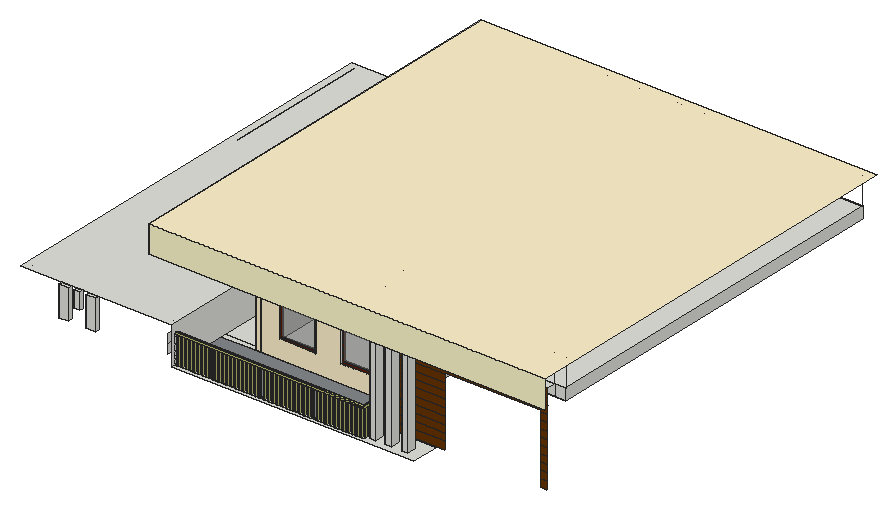
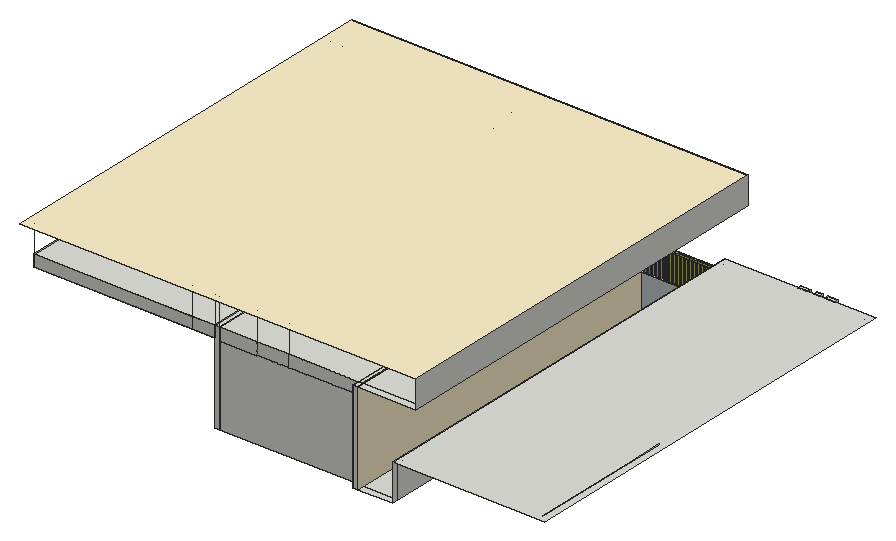
# SketchUp Ruby script. Lengths in inches.
U = 1.inch
M = Sketchup.active_model
def pt(a) = Geom::Point3d.new(a.map { |v| v * U })
def face(e, loops, mat)
  f = e.add_face(loops[0].map { |a| pt(a) })
  loops[1..].each { |l| e.add_face(l.map { |a| pt(a) }).erase! }
  f.material = f.back_material = mat if mat
  f
end
# faces: each face lists its corners as indices into pts; further lists are holes
def faces(e, pts, list, mat = nil) = list.each { |f| face(e, (f[0].is_a?(Array) ? f : [f]).map { |l| l.map { |i| pts[i] } }, mat) }
# xy, xz, yz: faces in a plane at the given z, y or x. An outline is a flat list of corners, or four numbers for a rectangle; further outlines are holes
def ring(l) = l.size == 4 ? [[l[0], l[1]], [l[2], l[1]], [l[2], l[3]], [l[0], l[3]]] : l.each_slice(2).to_a
def flat(e, list, mat, &to3) = list.each { |f| face(e, (f[0].is_a?(Array) ? f : [f]).map { |l| ring(l).map { |u, v| to3.(u, v) } }, mat) }
def xy(e, z, list, mat = nil) = flat(e, list, mat) { |x, y| [x, y, z] }
def xz(e, y, list, mat = nil) = flat(e, list, mat) { |x, z| [x, y, z] }
def yz(e, x, list, mat = nil) = flat(e, list, mat) { |y, z| [x, y, z] }
def lines(e, pts, list) = list.each { |a, b| e.add_line(pt(pts[a]), pt(pts[b])) }
# prism: a flat outline (further loops are holes) pulled along v
def prism(e, loops, v, mat = nil)
  f = face(e, loops, mat); d = Geom::Vector3d.new(v.map { |x| x * U })
  f.pushpull(f.normal.samedirection?(d) ? d.length : -d.length)
end
def box(e, o, s, mat = nil) = prism(e, [[o, [o[0] + s[0], o[1], o[2]], [o[0] + s[0], o[1] + s[1], o[2]], [o[0], o[1] + s[1], o[2]]]], [0, 0, s[2]], mat)
def at(x, y, z, deg = 0) = Geom::Transformation.translation(pt([x, y, z])) * Geom::Transformation.rotation(ORIGIN, Z_AXIS, deg.degrees)
def axes(o, x, y, z) = Geom::Transformation.new([*x, 0, *y, 0, *z, 0, *pt(o).to_a, 1])
def part(name) = M.definitions.add(name)
# library, detail: a bought-in or finely detailed component or shape, given as its bounding box
def library(name, o, s) = part(name).tap { |d| box(d.entities, o, s) }
def detail(e, o, s) = box(e.add_group.entities, o, s)
def put(e, d, t, mat = nil) = e.add_instance(d, t).tap { |i| i.material = mat if mat }
def group(e, t, mat = nil) = e.add_group.tap { |g| g.transformation = t; g.material = mat if mat }.entities
root = M.entities
M.materials.add("[0050_LemonChiffon]").color = [255, 250, 205]
M.materials.add("[Blacktop Old 01]").color = [132, 136, 139]
M.materials.add("[Color B08]").color = [102, 25, 0]
M.materials.add("[Color C08]").color = [102, 51, 0]
M.materials.add("[Color D01]").color = [255, 242, 204]
M.materials.add("[Metal Corrugated Shiny]").color = [193, 193, 113]
M.materials.add("[Translucent Glass Gray]").color = [128, 128, 128]
M.materials["[Translucent Glass Gray]"].alpha = 0.5
c1 = part("Group\#3")
xy(c1.entities,0,[[0,0,43.875,1.8125],[0,1.8125,43.875,3.875]],"[Color B08]")
xy(c1.entities,1.78,[[1.78,0,42.09,1.8125],[1.78,1.8125,42.09,3.875]],"[Color B08]")
xy(c1.entities,69.21,[[1.78,0,42.09,1.8125],[1.78,1.8125,42.09,3.875]],"[Color B08]")
xy(c1.entities,70.99,[[0,0,43.875,1.8125],[0,1.8125,43.875,3.875]],"[Color B08]")
xz(c1.entities,0,[[[0,0,43.875,70.99],[1.78,1.78,42.09,69.21]]],"[Color B08]")
xz(c1.entities,1.8125,[[[0,0,43.875,70.99],[1.78,1.78,42.09,69.21]]],"[Color B08]")
xz(c1.entities,1.8125,[[1.78,1.78,42.09,69.21]],"[Translucent Glass Gray]")
xz(c1.entities,3.875,[[[0,0,43.875,70.99],[1.78,1.78,42.09,69.21]]],"[Color B08]")
yz(c1.entities,0,[[0,0,1.8125,70.99],[1.8125,0,3.875,70.99]],"[Color B08]")
yz(c1.entities,1.78,[[0,1.78,1.8125,69.21],[1.8125,1.78,3.875,69.21]],"[Color B08]")
yz(c1.entities,42.09,[[0,1.78,1.8125,69.21],[1.8125,1.78,3.875,69.21]],"[Color B08]")
yz(c1.entities,43.875,[[0,0,1.8125,70.99],[1.8125,0,3.875,70.99]],"[Color B08]")
xy(root,496,[[[197.5625,128.625,512.0625,128.625,512.0625,165,444.53,165,444.53,132.625,197.5625,132.625],[488.28,138.19,497.22,149.57],[466.72,138.19,475.65,149.57],[446.72,138.19,455.65,149.57]],[[197.5625,132.625,444.53,132.625,444.53,165,441.53,165,441.53,135.625,197.5625,135.625],[441.94,136.33,444.17,137.7],[441.94,140.33,444.17,141.7],[441.94,144.33,444.17,145.7],[441.94,148.33,444.17,149.7],[441.94,152.33,444.17,153.7],[441.94,156.76,444.17,158.14],[441.94,162.45,444.17,163.83],[200.46,133.42,202.34,134.92],[205.77,133.42,207.65,134.92],[211.09,133.42,212.96,134.92],[216.4,133.42,218.27,134.92],[221.71,133.42,223.59,134.92],[227.02,133.42,228.9,134.92],[232.34,133.42,234.21,134.92],[237.65,133.42,239.52,134.92],[242.96,133.42,244.84,134.92],[248.27,133.42,250.15,134.92],[253.59,133.42,255.46,134.92],[258.9,133.42,260.77,134.92],[264.21,133.42,266.09,134.92],[269.52,133.42,271.4,134.92],[274.84,133.42,276.71,134.92],[280.15,133.42,282.02,134.92],[285.46,133.42,287.34,134.92],[290.77,133.42,292.65,134.92],[296.09,133.42,297.96,134.92],[301.4,133.42,303.27,134.92],[306.71,133.42,308.59,134.92],[312.46,133.42,314.34,134.92],[318.21,133.42,320.09,134.92],[323.96,133.42,325.84,134.92],[329.71,133.42,331.59,134.92],[335.46,133.42,337.34,134.92],[341.21,133.42,343.09,134.92],[346.96,133.42,348.84,134.92],[352.71,133.42,354.59,134.92],[358.46,133.42,360.34,134.92],[364.21,133.42,366.09,134.92],[369.96,133.42,371.84,134.92],[375.71,133.42,377.59,134.92],[381.46,133.42,383.34,134.92],[387.21,133.42,389.09,134.92],[392.96,133.42,394.84,134.92],[398.71,133.42,400.59,134.92],[404.46,133.42,406.34,134.92],[410.21,133.42,412.09,134.92],[415.96,133.42,417.84,134.92],[421.71,133.42,423.59,134.92],[427.46,133.42,429.34,134.92],[433.21,133.42,435.09,134.92],[438.96,133.42,440.84,134.92]],[197.5625,208.0625,243,214.0625],[243,208.0625,249,214.0625],[197.5625,214.0625,243,659.625],
  [243,214.0625,249,659.625],[249,214.0625,429.93,659.625],[197.5625,659.625,243,668.625],[243,659.625,249,668.625]])
xy(root,496,[[197.5625,135.625,441.53,135.625,441.53,165,430.125,165,430.125,208.0625,197.5625,208.0625]],"[Blacktop Old 01]")
xy(root,496,[[205.77,133.42,207.65,134.92],[211.09,133.42,212.96,134.92],[216.4,133.42,218.27,134.92],[221.71,133.42,223.59,134.92],[227.02,133.42,228.9,134.92],
  [232.34,133.42,234.21,134.92],[237.65,133.42,239.52,134.92],[242.96,133.42,244.84,134.92],[248.27,133.42,250.15,134.92],[253.59,133.42,255.46,134.92],
  [258.9,133.42,260.77,134.92],[264.21,133.42,266.09,134.92],[269.52,133.42,271.4,134.92],[274.84,133.42,276.71,134.92],[280.15,133.42,282.02,134.92],
  [285.46,133.42,287.34,134.92],[290.77,133.42,292.65,134.92],[296.09,133.42,297.96,134.92],[301.4,133.42,303.27,134.92],[306.71,133.42,308.59,134.92],
  [312.46,133.42,314.34,134.92],[318.21,133.42,320.09,134.92],[323.96,133.42,325.84,134.92],[329.71,133.42,331.59,134.92],[335.46,133.42,337.34,134.92],
  [341.21,133.42,343.09,134.92],[346.96,133.42,348.84,134.92],[352.71,133.42,354.59,134.92],[358.46,133.42,360.34,134.92],[364.21,133.42,366.09,134.92],
  [369.96,133.42,371.84,134.92],[375.71,133.42,377.59,134.92],[381.46,133.42,383.34,134.92],[387.21,133.42,389.09,134.92],[392.96,133.42,394.84,134.92],
  [398.71,133.42,400.59,134.92],[404.46,133.42,406.34,134.92],[410.21,133.42,412.09,134.92],[415.96,133.42,417.84,134.92],[421.71,133.42,423.59,134.92],
  [427.46,133.42,429.34,134.92],[433.21,133.42,435.09,134.92],[438.96,133.42,440.84,134.92],[441.94,136.33,444.17,137.7],[441.94,140.33,444.17,141.7],
  [441.94,144.33,444.17,145.7],[441.94,148.33,444.17,149.7],[441.94,152.33,444.17,153.7],[441.94,156.76,444.17,158.14],[441.94,162.45,444.17,163.83]],"[Metal Corrugated Shiny]")
xy(root,504.9375,[[54.48,123.625,66.79,128.625],[89.6,123.625,101.91,128.625]])
xy(root,519.5,[[273.67,208.0625,321.11,214.0625],[354.23,208.0625,401.67,214.0625]])
xy(root,522.8125,[[73.73,123.625,81.29,128.625]])
xy(root,532,[[[197.5625,132.625,441.53,135.625],[200.46,133.42,202.34,134.92],[205.77,133.42,207.65,134.92],[211.09,133.42,212.96,134.92],[216.4,133.42,218.27,134.92],[221.71,133.42,223.59,134.92],[227.02,133.42,228.9,134.92],[232.34,133.42,234.21,134.92],[237.65,133.42,239.52,134.92],[242.96,133.42,244.84,134.92],[248.27,133.42,250.15,134.92],[253.59,133.42,255.46,134.92],[258.9,133.42,260.77,134.92],[264.21,133.42,266.09,134.92],[269.52,133.42,271.4,134.92],[274.84,133.42,276.71,134.92],[280.15,133.42,282.02,134.92],[285.46,133.42,287.34,134.92],[290.77,133.42,292.65,134.92],[296.09,133.42,297.96,134.92],[301.4,133.42,303.27,134.92],[306.71,133.42,308.59,134.92],[312.46,133.42,314.34,134.92],[318.21,133.42,320.09,134.92],[323.96,133.42,325.84,134.92],[329.71,133.42,331.59,134.92],[335.46,133.42,337.34,134.92],[341.21,133.42,343.09,134.92],[346.96,133.42,348.84,134.92],[352.71,133.42,354.59,134.92],[358.46,133.42,360.34,134.92],[364.21,133.42,366.09,134.92],[369.96,133.42,371.84,134.92],[375.71,133.42,377.59,134.92],[381.46,133.42,383.34,134.92],[387.21,133.42,389.09,134.92],[392.96,133.42,394.84,134.92],[398.71,133.42,400.59,134.92],[404.46,133.42,406.34,134.92],[410.21,133.42,412.09,134.92],[415.96,133.42,417.84,134.92],[421.71,133.42,423.59,134.92],[427.46,133.42,429.34,134.92],[433.21,133.42,435.09,134.92],[438.96,133.42,440.84,134.92]],[[441.53,132.625,444.53,165],[441.94,136.33,444.17,137.7],[441.94,140.33,444.17,141.7],[441.94,144.33,444.17,145.7],[441.94,148.33,444.17,149.7],[441.94,152.33,444.17,153.7],[441.94,156.76,444.17,158.14],[441.94,162.45,444.17,163.83]]],"[Metal Corrugated Shiny]")
xy(root,534,[[197.5625,132.625,444.53,132.625,444.53,165,441.53,165,441.53,135.625,197.5625,135.625]],"[Metal Corrugated Shiny]")
xy(root,538,[[9,137.625,191.5625,659.625]])
xy(root,544,[[54.48,123.625,66.79,128.625],[73.73,123.625,81.29,128.625],[89.6,123.625,101.91,128.625],[0,128.625,197.5625,668.625]])
xy(root,587.25,[[523.3,165,648.11,177.0625]])
xy(root,596.26,[[273.67,208.0625,321.11,214.0625],[354.23,208.0625,401.67,214.0625]])
xy(root,599.8125,[[249,214.0625,429.93,659.625]])
xy(root,601.3125,[[436.125,177.0625,671.25,659.625]])
xy(root,616,[[[167.125,128.625,167.125,659.625,243,659.625,243,208.0625,430.125,208.0625,430.125,165,656.59,165,656.59,128.625],[446.72,138.19,455.65,149.57],[466.72,138.19,475.65,149.57],[488.28,138.19,497.22,149.57]],[446.72,138.19,455.65,149.57],[466.72,138.19,475.65,149.57],[488.28,138.19,497.22,149.57],[430.125,165,430.125,208.0625,249,208.0625,249,214.0625,436.125,214.0625,436.125,177.0625,656.59,177.0625,656.59,165],
  [436.125,177.0625,671.25,659.625],[243,208.0625,249,214.0625],[243,214.0625,249,659.625],[249,214.0625,429.93,659.625],[429.93,214.0625,436.125,659.625],
  [167.125,659.625,243,668.625],[243,659.625,249,668.625]])
xy(root,652,[[167.125,128.625,682.125,668.625]],"[Color D01]")
xz(root,123.625,[[54.48,504.9375,66.79,544],[89.6,504.9375,101.91,544],[73.73,522.8125,81.29,544]])
xz(root,128.625,[[54.48,504.9375,66.79,544],[89.6,504.9375,101.91,544],[73.73,522.8125,81.29,544]])
xz(root,128.625,[[167.125,616,682.125,652]],"[0050_LemonChiffon]")
xz(root,132.625,[[197.5625,532,444.53,534]],"[Metal Corrugated Shiny]")
xz(root,133.42,[[200.46,496,202.34,532],[205.77,496,207.65,532],[211.09,496,212.96,532],[216.4,496,218.27,532],[221.71,496,223.59,532],
  [227.02,496,228.9,532],[232.34,496,234.21,532],[237.65,496,239.52,532],[242.96,496,244.84,532],[248.27,496,250.15,532],
  [253.59,496,255.46,532],[258.9,496,260.77,532],[264.21,496,266.09,532],[269.52,496,271.4,532],[274.84,496,276.71,532],
  [280.15,496,282.02,532],[285.46,496,287.34,532],[290.77,496,292.65,532],[296.09,496,297.96,532],[301.4,496,303.27,532],
  [306.71,496,308.59,532],[312.46,496,314.34,532],[318.21,496,320.09,532],[323.96,496,325.84,532],[329.71,496,331.59,532],
  [335.46,496,337.34,532],[341.21,496,343.09,532],[346.96,496,348.84,532],[352.71,496,354.59,532],[358.46,496,360.34,532],
  [364.21,496,366.09,532],[369.96,496,371.84,532],[375.71,496,377.59,532],[381.46,496,383.34,532],[387.21,496,389.09,532],
  [392.96,496,394.84,532],[398.71,496,400.59,532],[404.46,496,406.34,532],[410.21,496,412.09,532],[415.96,496,417.84,532],
  [421.71,496,423.59,532],[427.46,496,429.34,532],[433.21,496,435.09,532],[438.96,496,440.84,532]],"[Metal Corrugated Shiny]")
xz(root,134.92,[[200.46,496,202.34,532],[205.77,496,207.65,532],[211.09,496,212.96,532],[216.4,496,218.27,532],[221.71,496,223.59,532],
  [227.02,496,228.9,532],[232.34,496,234.21,532],[237.65,496,239.52,532],[242.96,496,244.84,532],[248.27,496,250.15,532],
  [253.59,496,255.46,532],[258.9,496,260.77,532],[264.21,496,266.09,532],[269.52,496,271.4,532],[274.84,496,276.71,532],
  [280.15,496,282.02,532],[285.46,496,287.34,532],[290.77,496,292.65,532],[296.09,496,297.96,532],[301.4,496,303.27,532],
  [306.71,496,308.59,532],[312.46,496,314.34,532],[318.21,496,320.09,532],[323.96,496,325.84,532],[329.71,496,331.59,532],
  [335.46,496,337.34,532],[341.21,496,343.09,532],[346.96,496,348.84,532],[352.71,496,354.59,532],[358.46,496,360.34,532],
  [364.21,496,366.09,532],[369.96,496,371.84,532],[375.71,496,377.59,532],[381.46,496,383.34,532],[387.21,496,389.09,532],
  [392.96,496,394.84,532],[398.71,496,400.59,532],[404.46,496,406.34,532],[410.21,496,412.09,532],[415.96,496,417.84,532],
  [421.71,496,423.59,532],[427.46,496,429.34,532],[433.21,496,435.09,532],[438.96,496,440.84,532]],"[Metal Corrugated Shiny]")
xz(root,135.625,[[197.5625,532,441.53,534]],"[Metal Corrugated Shiny]")
xz(root,136.33,[[441.94,496,444.17,532]],"[Metal Corrugated Shiny]")
xz(root,137.7,[[441.94,496,444.17,532]],"[Metal Corrugated Shiny]")
xz(root,138.19,[[446.72,496,455.65,616],[466.72,496,475.65,616],[488.28,496,497.22,616]])
xz(root,140.33,[[441.94,496,444.17,532]],"[Metal Corrugated Shiny]")
xz(root,141.7,[[441.94,496,444.17,532]],"[Metal Corrugated Shiny]")
xz(root,144.33,[[441.94,496,444.17,532]],"[Metal Corrugated Shiny]")
xz(root,145.7,[[441.94,496,444.17,532]],"[Metal Corrugated Shiny]")
xz(root,148.33,[[441.94,496,444.17,532]],"[Metal Corrugated Shiny]")
xz(root,149.57,[[446.72,496,455.65,616],[466.72,496,475.65,616],[488.28,496,497.22,616]])
xz(root,149.7,[[441.94,496,444.17,532]],"[Metal Corrugated Shiny]")
xz(root,152.33,[[441.94,496,444.17,532]],"[Metal Corrugated Shiny]")
xz(root,153.7,[[441.94,496,444.17,532]],"[Metal Corrugated Shiny]")
xz(root,156.76,[[441.94,496,444.17,532]],"[Metal Corrugated Shiny]")
xz(root,158.14,[[441.94,496,444.17,532]],"[Metal Corrugated Shiny]")
xz(root,162.45,[[441.94,496,444.17,532]],"[Metal Corrugated Shiny]")
xz(root,163.83,[[441.94,496,444.17,532]],"[Metal Corrugated Shiny]")
xz(root,165,[[430.125,496,441.53,497.6],[441.53,496,444.53,532],[430.125,497.6,441.53,507.35],[430.125,507.35,441.53,517.1],[430.125,517.1,441.53,526.85],
  [441.53,532,444.53,534]])
xz(root,165,[[444.53,497.6,523.3,507.35],[648.11,497.6,656.59,507.35],[444.53,507.35,523.3,517.1],[648.11,507.35,656.59,517.1],[444.53,517.1,523.3,526.85],
  [648.11,517.1,656.59,526.85],[430.125,526.85,441.53,526.85,441.53,534,444.53,534,444.53,526.85,523.3,526.85,523.3,536.6,430.125,536.6],[648.11,526.85,656.59,536.6],[430.125,536.6,523.3,546.35],[648.11,536.6,656.59,546.35],
  [430.125,546.35,523.3,556.1],[648.11,546.35,656.59,556.1],[430.125,556.1,523.3,565.85],[648.11,556.1,656.59,565.85],[430.125,565.85,523.3,575.6],
  [648.11,565.85,656.59,575.6],[430.125,575.6,523.3,585.35],[648.11,575.6,656.59,585.35],[430.125,585.35,523.3,585.35,523.3,587.25,648.11,587.25,648.11,585.35,656.59,585.35,656.59,595.1,430.125,595.1],[430.125,595.1,656.59,604.85],
  [430.125,604.85,656.59,616]],"[Color C08]")
xz(root,177.0625,[[436.125,601.3125,656.59,616],[656.59,601.3125,671.25,616]])
xz(root,208.0625,[[243,496,249,616],[[249,496,430.125,616],[273.67,519.5,321.11,596.26],[354.23,519.5,401.67,596.26]]],"[Color D01]")
xz(root,214.0625,[[[249,496,429.93,599.8125],[273.67,519.5,321.11,596.26],[354.23,519.5,401.67,596.26]],[249,599.8125,429.93,616]])
xz(root,659.625,[[249,496,429.93,599.8125],[429.93,496,436.125,616],[249,599.8125,339.46,616],[339.46,599.8125,381.15,616],[381.15,599.8125,429.93,616],
  [436.125,601.3125,465,616],[465,601.3125,671.25,616]])
xz(root,668.625,[[243,496,249,616]])
yz(root,9,[[470.43,538,521.87,544],[521.87,538,659.625,544]])
yz(root,54.48,[[123.625,504.9375,128.625,544]])
yz(root,66.79,[[123.625,504.9375,128.625,544]])
yz(root,73.73,[[123.625,522.8125,128.625,544]])
yz(root,81.29,[[123.625,522.8125,128.625,544]])
yz(root,89.6,[[123.625,504.9375,128.625,544]])
yz(root,101.91,[[123.625,504.9375,128.625,544]])
yz(root,167.125,[[128.625,616,668.625,652]])
yz(root,191.5625,[[128.625,508,137.625,520],[128.625,520,137.625,532]])
yz(root,197.5625,[[128.625,496,132.625,496,132.625,534,135.625,534,135.625,496,659.625,496,659.625,544,128.625,544],[132.625,496,135.625,532],[659.625,496,668.625,544],[132.625,532,135.625,534]])
yz(root,200.46,[[133.42,496,134.92,532]],"[Metal Corrugated Shiny]")
yz(root,202.34,[[133.42,496,134.92,532]],"[Metal Corrugated Shiny]")
yz(root,205.77,[[133.42,496,134.92,532]],"[Metal Corrugated Shiny]")
yz(root,207.65,[[133.42,496,134.92,532]],"[Metal Corrugated Shiny]")
yz(root,211.09,[[133.42,496,134.92,532]],"[Metal Corrugated Shiny]")
yz(root,212.96,[[133.42,496,134.92,532]],"[Metal Corrugated Shiny]")
yz(root,216.4,[[133.42,496,134.92,532]],"[Metal Corrugated Shiny]")
yz(root,218.27,[[133.42,496,134.92,532]],"[Metal Corrugated Shiny]")
yz(root,221.71,[[133.42,496,134.92,532]],"[Metal Corrugated Shiny]")
yz(root,223.59,[[133.42,496,134.92,532]],"[Metal Corrugated Shiny]")
yz(root,227.02,[[133.42,496,134.92,532]],"[Metal Corrugated Shiny]")
yz(root,228.9,[[133.42,496,134.92,532]],"[Metal Corrugated Shiny]")
yz(root,232.34,[[133.42,496,134.92,532]],"[Metal Corrugated Shiny]")
yz(root,234.21,[[133.42,496,134.92,532]],"[Metal Corrugated Shiny]")
yz(root,237.65,[[133.42,496,134.92,532]],"[Metal Corrugated Shiny]")
yz(root,239.52,[[133.42,496,134.92,532]],"[Metal Corrugated Shiny]")
yz(root,242.96,[[133.42,496,134.92,532]],"[Metal Corrugated Shiny]")
yz(root,243,[[208.0625,496,668.625,616]],"[Color D01]")
yz(root,244.84,[[133.42,496,134.92,532]],"[Metal Corrugated Shiny]")
yz(root,248.27,[[133.42,496,134.92,532]],"[Metal Corrugated Shiny]")
yz(root,249,[[208.0625,496,214.0625,616],[214.0625,496,659.625,599.8125],[659.625,496,668.625,616],[214.0625,599.8125,659.625,616]])
yz(root,250.15,[[133.42,496,134.92,532]],"[Metal Corrugated Shiny]")
yz(root,253.59,[[133.42,496,134.92,532]],"[Metal Corrugated Shiny]")
yz(root,255.46,[[133.42,496,134.92,532]],"[Metal Corrugated Shiny]")
yz(root,258.9,[[133.42,496,134.92,532]],"[Metal Corrugated Shiny]")
yz(root,260.77,[[133.42,496,134.92,532]],"[Metal Corrugated Shiny]")
yz(root,264.21,[[133.42,496,134.92,532]],"[Metal Corrugated Shiny]")
yz(root,266.09,[[133.42,496,134.92,532]],"[Metal Corrugated Shiny]")
yz(root,269.52,[[133.42,496,134.92,532]],"[Metal Corrugated Shiny]")
yz(root,271.4,[[133.42,496,134.92,532]],"[Metal Corrugated Shiny]")
yz(root,273.67,[[208.0625,519.5,214.0625,596.26]])
yz(root,274.84,[[133.42,496,134.92,532]],"[Metal Corrugated Shiny]")
yz(root,276.71,[[133.42,496,134.92,532]],"[Metal Corrugated Shiny]")
yz(root,280.15,[[133.42,496,134.92,532]],"[Metal Corrugated Shiny]")
yz(root,282.02,[[133.42,496,134.92,532]],"[Metal Corrugated Shiny]")
yz(root,285.46,[[133.42,496,134.92,532]],"[Metal Corrugated Shiny]")
yz(root,287.34,[[133.42,496,134.92,532]],"[Metal Corrugated Shiny]")
yz(root,290.77,[[133.42,496,134.92,532]],"[Metal Corrugated Shiny]")
yz(root,292.65,[[133.42,496,134.92,532]],"[Metal Corrugated Shiny]")
yz(root,296.09,[[133.42,496,134.92,532]],"[Metal Corrugated Shiny]")
yz(root,297.96,[[133.42,496,134.92,532]],"[Metal Corrugated Shiny]")
yz(root,301.4,[[133.42,496,134.92,532]],"[Metal Corrugated Shiny]")
yz(root,303.27,[[133.42,496,134.92,532]],"[Metal Corrugated Shiny]")
yz(root,306.71,[[133.42,496,134.92,532]],"[Metal Corrugated Shiny]")
yz(root,308.59,[[133.42,496,134.92,532]],"[Metal Corrugated Shiny]")
yz(root,312.46,[[133.42,496,134.92,532]],"[Metal Corrugated Shiny]")
yz(root,314.34,[[133.42,496,134.92,532]],"[Metal Corrugated Shiny]")
yz(root,318.21,[[133.42,496,134.92,532]],"[Metal Corrugated Shiny]")
yz(root,320.09,[[133.42,496,134.92,532]],"[Metal Corrugated Shiny]")
yz(root,321.11,[[208.0625,519.5,214.0625,596.26]])
yz(root,323.96,[[133.42,496,134.92,532]],"[Metal Corrugated Shiny]")
yz(root,325.84,[[133.42,496,134.92,532]],"[Metal Corrugated Shiny]")
yz(root,329.71,[[133.42,496,134.92,532]],"[Metal Corrugated Shiny]")
yz(root,331.59,[[133.42,496,134.92,532]],"[Metal Corrugated Shiny]")
yz(root,335.46,[[133.42,496,134.92,532]],"[Metal Corrugated Shiny]")
yz(root,337.34,[[133.42,496,134.92,532]],"[Metal Corrugated Shiny]")
yz(root,341.21,[[133.42,496,134.92,532]],"[Metal Corrugated Shiny]")
yz(root,343.09,[[133.42,496,134.92,532]],"[Metal Corrugated Shiny]")
yz(root,346.96,[[133.42,496,134.92,532]],"[Metal Corrugated Shiny]")
yz(root,348.84,[[133.42,496,134.92,532]],"[Metal Corrugated Shiny]")
yz(root,352.71,[[133.42,496,134.92,532]],"[Metal Corrugated Shiny]")
yz(root,354.23,[[208.0625,519.5,214.0625,596.26]])
yz(root,354.59,[[133.42,496,134.92,532]],"[Metal Corrugated Shiny]")
yz(root,358.46,[[133.42,496,134.92,532]],"[Metal Corrugated Shiny]")
yz(root,360.34,[[133.42,496,134.92,532]],"[Metal Corrugated Shiny]")
yz(root,364.21,[[133.42,496,134.92,532]],"[Metal Corrugated Shiny]")
yz(root,366.09,[[133.42,496,134.92,532]],"[Metal Corrugated Shiny]")
yz(root,369.96,[[133.42,496,134.92,532]],"[Metal Corrugated Shiny]")
yz(root,371.84,[[133.42,496,134.92,532]],"[Metal Corrugated Shiny]")
yz(root,375.71,[[133.42,496,134.92,532]],"[Metal Corrugated Shiny]")
yz(root,377.59,[[133.42,496,134.92,532]],"[Metal Corrugated Shiny]")
yz(root,381.46,[[133.42,496,134.92,532]],"[Metal Corrugated Shiny]")
yz(root,383.34,[[133.42,496,134.92,532]],"[Metal Corrugated Shiny]")
yz(root,387.21,[[133.42,496,134.92,532]],"[Metal Corrugated Shiny]")
yz(root,389.09,[[133.42,496,134.92,532]],"[Metal Corrugated Shiny]")
yz(root,392.96,[[133.42,496,134.92,532]],"[Metal Corrugated Shiny]")
yz(root,394.84,[[133.42,496,134.92,532]],"[Metal Corrugated Shiny]")
yz(root,398.71,[[133.42,496,134.92,532]],"[Metal Corrugated Shiny]")
yz(root,400.59,[[133.42,496,134.92,532]],"[Metal Corrugated Shiny]")
yz(root,401.67,[[208.0625,519.5,214.0625,596.26]])
yz(root,404.46,[[133.42,496,134.92,532]],"[Metal Corrugated Shiny]")
yz(root,406.34,[[133.42,496,134.92,532]],"[Metal Corrugated Shiny]")
yz(root,410.21,[[133.42,496,134.92,532]],"[Metal Corrugated Shiny]")
yz(root,412.09,[[133.42,496,134.92,532]],"[Metal Corrugated Shiny]")
yz(root,415.96,[[133.42,496,134.92,532]],"[Metal Corrugated Shiny]")
yz(root,417.84,[[133.42,496,134.92,532]],"[Metal Corrugated Shiny]")
yz(root,421.71,[[133.42,496,134.92,532]],"[Metal Corrugated Shiny]")
yz(root,423.59,[[133.42,496,134.92,532]],"[Metal Corrugated Shiny]")
yz(root,427.46,[[133.42,496,134.92,532]],"[Metal Corrugated Shiny]")
yz(root,429.34,[[133.42,496,134.92,532]],"[Metal Corrugated Shiny]")
yz(root,429.93,[[214.0625,496,659.625,599.8125],[214.0625,599.8125,659.625,616]])
yz(root,430.125,[[165,496,208.0625,616]],"[Color C08]")
yz(root,433.21,[[133.42,496,134.92,532]],"[Metal Corrugated Shiny]")
yz(root,435.09,[[133.42,496,134.92,532]],"[Metal Corrugated Shiny]")
yz(root,436.125,[[177.0625,601.3125,214.0625,616],[214.0625,601.3125,659.625,616]])
yz(root,438.96,[[133.42,496,134.92,532]],"[Metal Corrugated Shiny]")
yz(root,440.84,[[133.42,496,134.92,532]],"[Metal Corrugated Shiny]")
yz(root,441.53,[[135.625,532,165,534]],"[Metal Corrugated Shiny]")
yz(root,441.94,[[136.33,496,137.7,532],[140.33,496,141.7,532],[144.33,496,145.7,532],[148.33,496,149.7,532],[152.33,496,153.7,532],
  [156.76,496,158.14,532],[162.45,496,163.83,532]],"[Metal Corrugated Shiny]")
yz(root,444.17,[[136.33,496,137.7,532],[140.33,496,141.7,532],[144.33,496,145.7,532],[148.33,496,149.7,532],[152.33,496,153.7,532],
  [156.76,496,158.14,532],[162.45,496,163.83,532]],"[Metal Corrugated Shiny]")
yz(root,444.53,[[132.625,532,165,534]],"[Metal Corrugated Shiny]")
yz(root,446.72,[[138.19,496,149.57,616]])
yz(root,455.65,[[138.19,496,149.57,616]])
yz(root,466.72,[[138.19,496,149.57,616]])
yz(root,475.65,[[138.19,496,149.57,616]])
yz(root,488.28,[[138.19,496,149.57,616]])
yz(root,497.22,[[138.19,496,149.57,616]])
yz(root,671.25,[[177.0625,601.3125,659.625,616]])
p = [[9,137.625,538],[9,137.625,544],[191.5625,659.625,538],[191.5625,659.625,544],[191.5625,137.625,538],[191.5625,137.625,544],
  [465,659.625,616],[465,659.625,652],[436.125,177.0625,616],[436.125,177.0625,652],[656.59,177.0625,616],[656.59,177.0625,652],
  [671.25,177.0625,616],[671.25,177.0625,652],[671.25,659.625,616],[671.25,659.625,652],[436.125,659.625,616],[436.125,659.625,652],
  [339.46,659.625,616],[339.46,659.625,652],[381.15,659.625,616],[381.15,659.625,652],[429.93,214.0625,616],[429.93,214.0625,652],
  [429.93,659.625,616],[429.93,659.625,652]]
lines(root,p,[[0,1],[2,3],[4,5],[6,7],[8,9],[10,11],[12,13],[14,15],[16,17],[18,19],[20,21],[22,23],
  [24,25]])
put(root,c1,axes([273.48,208.84,519.5],[1.08558,0,0],[0,0.8,0],[0,0,1.07971]))
put(root,c1,axes([354.04,208.84,519.5],[1.08558,0,0],[0,0.8,0],[0,0,1.07971]))
